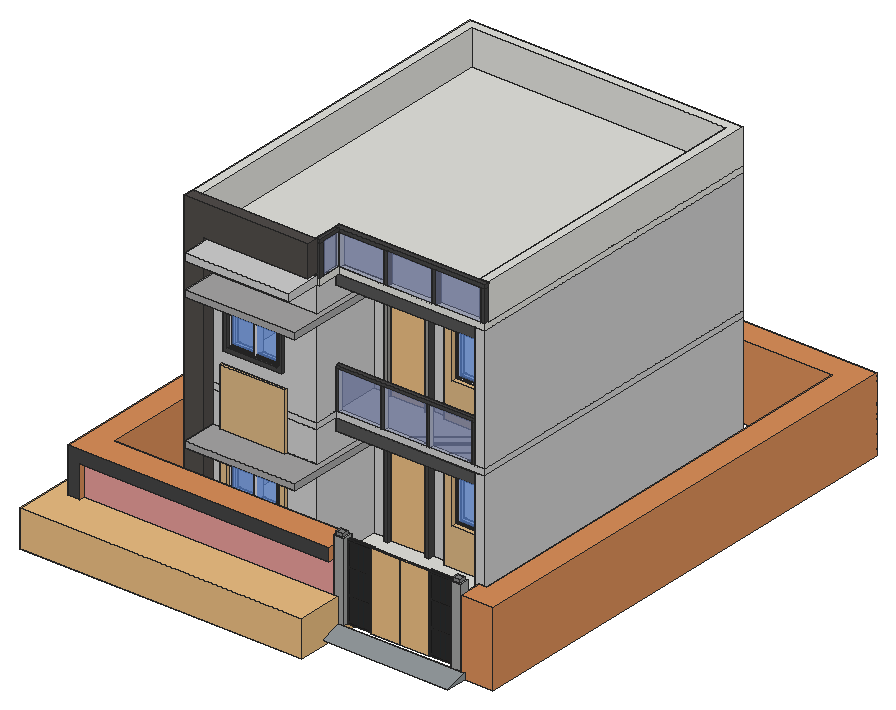
# SketchUp Ruby script. Lengths in inches.
U = 1.inch
M = Sketchup.active_model
def pt(a) = Geom::Point3d.new(a.map { |v| v * U })
def face(e, loops, mat)
  f = e.add_face(loops[0].map { |a| pt(a) })
  loops[1..].each { |l| e.add_face(l.map { |a| pt(a) }).erase! }
  f.material = f.back_material = mat if mat
  f
end
# faces: each face lists its corners as indices into pts; further lists are holes
def faces(e, pts, list, mat = nil) = list.each { |f| face(e, (f[0].is_a?(Array) ? f : [f]).map { |l| l.map { |i| pts[i] } }, mat) }
# xy, xz, yz: faces in a plane at the given z, y or x. An outline is a flat list of corners, or four numbers for a rectangle; further outlines are holes
def ring(l) = l.size == 4 ? [[l[0], l[1]], [l[2], l[1]], [l[2], l[3]], [l[0], l[3]]] : l.each_slice(2).to_a
def flat(e, list, mat, &to3) = list.each { |f| face(e, (f[0].is_a?(Array) ? f : [f]).map { |l| ring(l).map { |u, v| to3.(u, v) } }, mat) }
def xy(e, z, list, mat = nil) = flat(e, list, mat) { |x, y| [x, y, z] }
def xz(e, y, list, mat = nil) = flat(e, list, mat) { |x, z| [x, y, z] }
def yz(e, x, list, mat = nil) = flat(e, list, mat) { |y, z| [x, y, z] }
def lines(e, pts, list) = list.each { |a, b| e.add_line(pt(pts[a]), pt(pts[b])) }
# prism: a flat outline (further loops are holes) pulled along v
def prism(e, loops, v, mat = nil)
  f = face(e, loops, mat); d = Geom::Vector3d.new(v.map { |x| x * U })
  f.pushpull(f.normal.samedirection?(d) ? d.length : -d.length)
end
def box(e, o, s, mat = nil) = prism(e, [[o, [o[0] + s[0], o[1], o[2]], [o[0] + s[0], o[1] + s[1], o[2]], [o[0], o[1] + s[1], o[2]]]], [0, 0, s[2]], mat)
def at(x, y, z, deg = 0) = Geom::Transformation.translation(pt([x, y, z])) * Geom::Transformation.rotation(ORIGIN, Z_AXIS, deg.degrees)
def axes(o, x, y, z) = Geom::Transformation.new([*x, 0, *y, 0, *z, 0, *pt(o).to_a, 1])
def part(name) = M.definitions.add(name)
# library, detail: a bought-in or finely detailed component or shape, given as its bounding box
def library(name, o, s) = part(name).tap { |d| box(d.entities, o, s) }
def detail(e, o, s) = box(e.add_group.entities, o, s)
def put(e, d, t, mat = nil) = e.add_instance(d, t).tap { |i| i.material = mat if mat }
def group(e, t, mat = nil) = e.add_group.tap { |g| g.transformation = t; g.material = mat if mat }.entities
root = M.entities
M.materials.add("18776129-polished-granite-texture-in-whites-grays-and-blacks").color = [192, 192, 186]
M.materials.add("Lisanne_Eraser").color = [146, 152, 155]
M.materials.add("Stone_A_200cm").color = [133, 133, 133]
M.materials.add("Stone_A_200cmgach trang tri").color = [160, 161, 160]
M.materials.add("THEPDEN").color = [42, 49, 51]
M.materials.add("[Beadboard]").color = [218, 143, 90]
M.materials.add("[Brick Basket]").color = [230, 156, 152]
M.materials.add("[Carrera Marble]").color = [207, 207, 207]
M.materials.add("[Cladding Siding White]").color = [207, 207, 207]
M.materials.add("[Granite Dark Gray]").color = [69, 68, 68]
M.materials.add("[Granite Light Gray]").color = [149, 148, 144]
M.materials.add("[Metal Rusted]").color = [184, 117, 91]
M.materials.add("[Metal Silver]").color = [234, 233, 238]
M.materials.add("[Roofing Shingles GAF Estates]").color = [81, 77, 74]
M.materials.add("[Stone Vein Gray]").color = [166, 165, 165]
M.materials.add("[Suede Blue]").color = [50, 57, 70]
M.materials.add("[Suede Dark Gray]").color = [85, 85, 85]
M.materials.add("[Translucent Glass Blue]").color = [100, 149, 237]
M.materials["[Translucent Glass Blue]"].alpha = 0.5
M.materials.add("[Translucent Glass Sky Reflection]").color = [126, 138, 183]
M.materials["[Translucent Glass Sky Reflection]"].alpha = 0.52
M.materials.add("[Wallpaper Stripe]").color = [222, 185, 133]
M.materials.add("sat son den1").color = [33, 33, 33]
c1 = part("Component\#28")
box(c1.entities,[0,0,0],[7.875,7.875,3.9375],"Stone_A_200cm")
c2 = library("Group\#58",[-9.3,-11.72,-5.59],[177.13,38.12,35])
c3 = part("Vertical slat panel")
g1 = group(c3.entities,at(21.95,0,0))
box(g1,[0,0,0],[0.79,1.57,29.73],"THEPDEN")
g2 = group(c3.entities,at(5.49,0,0))
box(g2,[0,0,0],[0.79,1.57,29.73],"THEPDEN")
g3 = group(c3.entities,at(10.98,0,0))
box(g3,[0,0,0],[0.79,1.57,29.73],"THEPDEN")
g4 = group(c3.entities,at(7.84,0.79,0,-90))
box(g4,[0,0,0],[0.79,1.57,29.73],"THEPDEN")
g5 = group(c3.entities,at(13.33,0.79,0,-90))
box(g5,[0,0,0],[0.79,1.57,29.73],"THEPDEN")
g6 = group(c3.entities,at(2.35,0.79,0,-90))
box(g6,[0,0,0],[0.79,1.57,29.73],"THEPDEN")
g7 = group(c3.entities,at(18.8125,0.79,0,-90))
box(g7,[0,0,0],[0.79,1.57,29.73],"THEPDEN")
g8 = group(c3.entities,at(16.46,0,0))
box(g8,[0,0,0],[0.79,1.57,29.73],"THEPDEN")
g9 = group(c3.entities,at(24.3,0.79,0,-90))
box(g9,[0,0,0],[0.79,1.57,29.73],"THEPDEN")
c4 = part("Slatted gate leaf")
put(c4.entities,c3,axes([24.84,1.79,-51.33],[1.0302,0,0],[0,1,0],[0,0,0.84297]))
put(c4.entities,c3,axes([24.84,1.79,-104.14],[1.0302,0,0],[0,1,0],[0,0,0.82146]))
put(c4.entities,c3,axes([24.84,1.79,-78.28],[1.0302,0,0],[0,1,0],[0,0,0.8582]))
g10 = group(c4.entities,at(34.94,4.25,0))
xy(g10,-105.55,[[-10.84,-4.25,19.38,0]],"sat son den1")
xy(g10,-103.49,[[-8.39,-4.25,16.93,0]],"sat son den1")
xy(g10,-79.72,[[-9.2,-4.25,-8.39,0],[-8.39,-4.25,16.93,0],[16.93,-4.25,17.74,0]],"sat son den1")
xy(g10,-79.24,[[-10.37,-4.25,-9.2,0],[17.74,-4.25,18.92,0]],"sat son den1")
xy(g10,-78.77,[[-10.37,-4.25,-9.2,0],[17.74,-4.25,18.92,0]],"sat son den1")
xy(g10,-78.28,[[-9.2,-4.25,-8.39,0],[-8.39,-4.25,16.93,0],[16.93,-4.25,17.74,0]],"sat son den1")
xy(g10,-52.77,[[-9.2,-4.25,-8.39,0],[-8.39,-4.25,16.93,0],[16.93,-4.25,17.74,0]],"sat son den1")
xy(g10,-52.28,[[-10.37,-4.25,-9.2,0],[17.74,-4.25,18.92,0]],"sat son den1")
xy(g10,-51.82,[[-10.37,-4.25,-9.2,0],[17.74,-4.25,18.92,0]],"sat son den1")
xy(g10,-51.33,[[-9.2,-4.25,-8.39,0],[-8.39,-4.25,16.93,0],[16.93,-4.25,17.74,0]],"sat son den1")
xy(g10,-26.92,[[-8.39,-4.25,16.93,0]],"sat son den1")
xy(g10,-26.27,[[-10.37,-4.25,-8.39,0],[16.93,-4.25,17.74,0]],"sat son den1")
xy(g10,-25.33,[[17.74,-4.25,18.92,0]],"sat son den1")
xy(g10,-24.87,[[-10.84,-4.25,-10.37,0],[-10.37,-4.25,18.92,0],[18.92,-4.25,19.38,0]],"sat son den1")
xz(g10,-4.25,[[-10.84,-105.55,19.38,-105.55,19.38,-24.87,18.92,-24.87,18.92,-25.33,17.74,-25.33,17.74,-26.27,16.93,-26.27,16.93,-51.33,17.74,-51.33,17.74,-51.82,18.92,-51.82,18.92,-52.28,17.74,-52.28,17.74,-52.77,16.93,-52.77,16.93,-78.28,17.74,-78.28,17.74,-78.77,18.92,-78.77,18.92,-79.24,17.74,-79.24,17.74,-79.72,16.93,-79.72,16.93,-103.49,-8.39,-103.49,-8.39,-79.72,-9.2,-79.72,-9.2,-79.24,-10.37,-79.24,-10.37,-78.77,-9.2,-78.77,-9.2,-78.28,-8.39,-78.28,-8.39,-52.77,-9.2,-52.77,-9.2,-52.28,-10.37,-52.28,-10.37,-51.82,-9.2,-51.82,-9.2,-51.33,-8.39,-51.33,-8.39,-26.27,-10.37,-26.27,-10.37,-24.87,-10.84,-24.87],[-9.2,-79.72,17.74,-79.72,17.74,-79.24,18.92,-79.24,18.92,-78.77,17.74,-78.77,17.74,-78.28,-9.2,-78.28,-9.2,-78.77,-10.37,-78.77,-10.37,-79.24,-9.2,-79.24],[-9.2,-52.77,17.74,-52.77,17.74,-52.28,18.92,-52.28,18.92,-51.82,17.74,-51.82,17.74,-51.33,-9.2,-51.33,-9.2,-51.82,-10.37,-51.82,-10.37,-52.28,-9.2,-52.28],[-8.39,-26.92,16.93,-26.92,16.93,-26.27,17.74,-26.27,17.74,-25.33,18.92,-25.33,18.92,-24.87,-10.37,-24.87,-10.37,-26.27,-8.39,-26.27]],"sat son den1")
xz(g10,0,[[-10.84,-105.55,-10.84,-24.87,-10.37,-24.87,-10.37,-26.27,-8.39,-26.27,-8.39,-51.33,-9.2,-51.33,-9.2,-51.82,-10.37,-51.82,-10.37,-52.28,-9.2,-52.28,-9.2,-52.77,-8.39,-52.77,-8.39,-78.28,-9.2,-78.28,-9.2,-78.77,-10.37,-78.77,-10.37,-79.24,-9.2,-79.24,-9.2,-79.72,-8.39,-79.72,-8.39,-103.49,16.93,-103.49,16.93,-79.72,17.74,-79.72,17.74,-79.24,18.92,-79.24,18.92,-78.77,17.74,-78.77,17.74,-78.28,16.93,-78.28,16.93,-52.77,17.74,-52.77,17.74,-52.28,18.92,-52.28,18.92,-51.82,17.74,-51.82,17.74,-51.33,16.93,-51.33,16.93,-26.27,17.74,-26.27,17.74,-25.33,18.92,-25.33,18.92,-24.87,19.38,-24.87,19.38,-105.55],[-9.2,-79.72,-9.2,-79.24,-10.37,-79.24,-10.37,-78.77,-9.2,-78.77,-9.2,-78.28,17.74,-78.28,17.74,-78.77,18.92,-78.77,18.92,-79.24,17.74,-79.24,17.74,-79.72],[-9.2,-52.77,-9.2,-52.28,-10.37,-52.28,-10.37,-51.82,-9.2,-51.82,-9.2,-51.33,17.74,-51.33,17.74,-51.82,18.92,-51.82,18.92,-52.28,17.74,-52.28,17.74,-52.77],[-8.39,-26.92,-8.39,-26.27,-10.37,-26.27,-10.37,-24.87,18.92,-24.87,18.92,-25.33,17.74,-25.33,17.74,-26.27,16.93,-26.27,16.93,-26.92]],"sat son den1")
yz(g10,-10.84,[[-4.25,-105.55,0,-24.87]],"sat son den1")
yz(g10,-10.37,[[-4.25,-79.24,0,-78.77],[-4.25,-52.28,0,-51.82],[-4.25,-26.27,0,-24.87]],"sat son den1")
yz(g10,-9.2,[[-4.25,-79.72,0,-79.24],[-4.25,-78.77,0,-78.28],[-4.25,-52.77,0,-52.28],[-4.25,-51.82,0,-51.33]],"sat son den1")
yz(g10,-8.39,[[-4.25,-103.49,0,-79.72],[-4.25,-78.28,0,-52.77],[-4.25,-51.33,0,-26.92],[-4.25,-26.92,0,-26.27]],"sat son den1")
yz(g10,16.93,[[-4.25,-103.49,0,-79.72],[-4.25,-78.28,0,-52.77],[-4.25,-51.33,0,-26.92],[-4.25,-26.92,0,-26.27]],"sat son den1")
yz(g10,17.74,[[-4.25,-79.72,0,-79.24],[-4.25,-78.77,0,-78.28],[-4.25,-52.77,0,-52.28],[-4.25,-51.82,0,-51.33],[-4.25,-26.27,0,-25.33]],"sat son den1")
yz(g10,18.92,[[-4.25,-79.24,0,-78.77],[-4.25,-52.28,0,-51.82],[-4.25,-25.33,0,-24.87]],"sat son den1")
yz(g10,19.38,[[-4.25,-105.55,0,-24.87]],"sat son den1")
c5 = library("Group\#45",[0,-0.15,0],[31.47,2.91,94.32])
c6 = library("Group\#35",[0,-0.15,0],[31.47,2.91,94.32])
c7 = part("cong+trinh+1")
put(c7.entities,c1,axes([-761.28,-1219.33,75.2],[0.82267,0,0],[0,0.76,0],[0,0,0.75]))
put(c7.entities,c1,axes([-647.9,-1219.33,75.2],[0.82267,0,0],[0,0.76,0],[0,0,0.75]))
g11 = group(c7.entities,at(614.78,209.1,-17.8125))
g12 = group(g11,at(-1250.68,-1449.6,11.8125),"18776129-polished-granite-texture-in-whites-grays-and-blacks")
prism(g12,[[[-132.06,19.69,5.91],[-132.06,19.69,0],[-132.06,0,0]]],[132.06,0,0],"Lisanne_Eraser")
put(c7.entities,c2,axes([-1016.9,-1244.91,-6],[1.5402,0,0],[0,1.68,0],[0,0,1]))
g13 = group(c7.entities,at(-649.52,-1220.82,-0.09))
box(g13,[0,0,0],[9.72,8.98,75.3],"Stone_A_200cmgach trang tri")
g14 = group(c7.entities,at(-762.9,-1220.82,-0.09))
box(g14,[0,0,0],[9.72,8.98,75.3],"Stone_A_200cmgach trang tri")
g15 = group(c7.entities,at(-753.18,-1217.23,-0.09))
put(g15,c4,axes([60.26,3.95,-22.7],[0.79856,0,0],[0,-0.76,0],[0,0,-0.913]))
put(g15,c4,axes([-19.25,3.95,-22.7],[0.79856,0,0],[0,-0.76,0],[0,0,-0.913]))
put(g15,c5,axes([24.03,0.12,0],[0.88335,0,0],[0,0.76,0],[0,0,0.78261]),"THEPDEN")
put(g15,c6,axes([79.62,0.12,0],[-0.88335,0,0],[0,0.76,0],[0,0,0.78261]))
c8 = part("Group4\#2")
box(c8.entities,[1.02,-2.16,1.02],[46.66,0.63,45.96])
c9 = part("Group\#3")
g16 = group(c9.entities,at(48.7,0,0,180),"[Metal Silver]")
xy(g16,0,[[0,-9,23.52,0],[23.52,-9,25.18,0],[25.18,-9,48.7,0]])
xy(g16,0.83,[[0.83,-8.93,23.52,-4.61],[25.18,-8.93,47.875,-4.61]])
xy(g16,1.02,[[1.02,-3.3125,23.52,-2.16],[23.52,-3.3125,25.18,-2.16],[25.18,-3.3125,47.68,-2.16]])
xy(g16,1.61,[[1.61,-2.16,23.52,-1.8],[25.18,-2.16,47.09,-1.8]])
xy(g16,1.65,[[1.65,-3.46,23.52,-3.3125],[25.18,-3.46,47.05,-3.3125]])
xy(g16,46.35,[[1.65,-3.46,23.52,-3.3125],[25.18,-3.46,47.05,-3.3125]])
xy(g16,46.39,[[1.61,-2.16,23.52,-1.8],[25.18,-2.16,47.09,-1.8]])
xy(g16,46.98,[[1.02,-3.3125,23.52,-2.16],[23.52,-3.3125,25.18,-2.16],[25.18,-3.3125,47.68,-2.16]])
xy(g16,47.17,[[0.83,-8.93,23.52,-4.61],[25.18,-8.93,47.875,-4.61]])
xy(g16,48,[[0,-9,23.52,0],[23.52,-9,25.18,0],[25.18,-9,48.7,0]])
xz(g16,-9.07,[[0.04,0.04,23.52,0.04,23.52,0.75,0.75,0.75,0.75,47.25,23.52,47.25,23.52,47.96,0.04,47.96],[23.52,0.04,25.18,47.96],[25.18,0.04,48.66,0.04,48.66,47.96,25.18,47.96,25.18,47.25,47.95,47.25,47.95,0.75,25.18,0.75]])
xz(g16,-4.61,[[0.83,0.83,23.52,0.83,23.52,1.5,1.5,1.5,1.5,46.5,23.52,46.5,23.52,47.17,0.83,47.17],[25.18,0.83,47.875,0.83,47.875,47.17,25.18,47.17,25.18,46.5,47.21,46.5,47.21,1.5,25.18,1.5]])
xz(g16,-3.3125,[[1.02,1.02,1.02,46.98,23.52,46.98,23.52,46.35,1.65,46.35,1.65,1.65,23.52,1.65,23.52,1.02],[23.52,1.02,25.18,46.98],[25.18,1.02,25.18,1.65,47.05,1.65,47.05,46.35,25.18,46.35,25.18,46.98,47.68,46.98,47.68,1.02]])
xz(g16,-2.16,[[1.02,1.02,23.52,1.02,23.52,1.61,1.61,1.61,1.61,46.39,23.52,46.39,23.52,46.98,1.02,46.98],[23.52,1.02,25.18,46.98],[25.18,1.02,47.68,1.02,47.68,46.98,25.18,46.98,25.18,46.39,47.09,46.39,47.09,1.61,25.18,1.61]])
xz(g16,-1.8,[[0.83,0.83,0.83,47.17,23.52,47.17,23.52,46.39,1.61,46.39,1.61,1.61,23.52,1.61,23.52,0.83],[25.18,0.83,25.18,1.61,47.09,1.61,47.09,46.39,25.18,46.39,25.18,47.17,47.875,47.17,47.875,0.83]])
xz(g16,-0.36,[[0.59,0.59,0.59,47.41,23.52,47.41,23.52,47.21,0.79,47.21,0.79,0.79,23.52,0.79,23.52,0.59],[25.18,0.59,25.18,0.79,47.91,0.79,47.91,47.21,25.18,47.21,25.18,47.41,48.11,47.41,48.11,0.59]])
xz(g16,0,[[0,0,0,48,23.52,48,23.52,47.61,0.39,47.61,0.39,0.39,23.52,0.39,23.52,0],[23.52,0,25.18,48],[25.18,0,25.18,0.39,48.31,0.39,48.31,47.61,25.18,47.61,25.18,48,48.7,48,48.7,0]])
yz(g16,0,[[-9,0,0,48]])
yz(g16,0.83,[[-8.93,0.83,-4.61,47.17]])
yz(g16,1.02,[[-3.3125,1.02,-2.16,46.98]])
yz(g16,1.61,[[-2.16,1.61,-1.8,46.39]])
yz(g16,1.65,[[-3.46,1.65,-3.3125,46.35]])
yz(g16,23.52,[[-9,0,0,0,0,0.39,-0.36,0.59,-0.36,0.79,-1.8,0.83,-1.8,1.61,-2.16,1.61,-2.16,1.02,-3.3125,1.02,-3.3125,1.65,-3.46,1.65,-4.61,1.5,-4.61,0.83,-8.93,0.83,-9.07,0.75,-9.07,0.04],[[-9,0,-9.07,0.04,-9.07,47.96,-9,48,0,48,0,0],[-3.3125,1.02,-2.16,46.98]],[-3.46,46.35,-3.3125,46.35,-3.3125,46.98,-2.16,46.98,-2.16,46.39,-1.8,46.39,-1.8,47.17,-0.36,47.21,-0.36,47.41,0,47.61,0,48,-9,48,-9.07,47.96,-9.07,47.25,-8.93,47.17,-4.61,47.17,-4.61,46.5]])
yz(g16,25.18,[[-9,0,-9.07,0.04,-9.07,0.75,-8.93,0.83,-4.61,0.83,-4.61,1.5,-3.46,1.65,-3.3125,1.65,-3.3125,1.02,-2.16,1.02,-2.16,1.61,-1.8,1.61,-1.8,0.83,-0.36,0.79,-0.36,0.59,0,0.39,0,0],[[-9,0,0,0,0,48,-9,48,-9.07,47.96,-9.07,0.04],[-3.3125,1.02,-2.16,46.98]],[-3.46,46.35,-4.61,46.5,-4.61,47.17,-8.93,47.17,-9.07,47.25,-9.07,47.96,-9,48,0,48,0,47.61,-0.36,47.41,-0.36,47.21,-1.8,47.17,-1.8,46.39,-2.16,46.39,-2.16,46.98,-3.3125,46.98,-3.3125,46.35]])
yz(g16,47.05,[[-3.46,1.65,-3.3125,46.35]])
yz(g16,47.09,[[-2.16,1.61,-1.8,46.39]])
yz(g16,47.68,[[-3.3125,1.02,-2.16,46.98]])
yz(g16,47.875,[[-8.93,0.83,-4.61,47.17]])
yz(g16,48.7,[[-9,0,0,48]])
p = [[23.52,-9,0],[23.52,-9.07,0.04],[0.04,-9.07,0.04],[0,-9,0],[0.04,-9.07,47.96],[0,-9,48],
  [25.18,-9,0],[25.18,-9.07,0.04],[48.7,-9,0],[48.66,-9.07,0.04],[48.7,-9,48],[48.66,-9.07,47.96],
  [23.52,-0.36,0.59],[23.52,0,0.39],[0.39,0,0.39],[0.59,-0.36,0.59],[0.39,0,47.61],[0.59,-0.36,47.41],
  [25.18,0,0.39],[25.18,-0.36,0.59],[48.11,-0.36,0.59],[48.31,0,0.39],[48.11,-0.36,47.41],[48.31,0,47.61],
  [23.52,-9.07,0.75],[23.52,-8.93,0.83],[0.83,-8.93,0.83],[0.75,-9.07,0.75],[0.83,-8.93,47.17],[0.75,-9.07,47.25],
  [25.18,-8.93,0.83],[25.18,-9.07,0.75],[47.95,-9.07,0.75],[47.875,-8.93,0.83],[47.95,-9.07,47.25],[47.875,-8.93,47.17],
  [23.52,-1.8,0.83],[23.52,-0.36,0.79],[0.79,-0.36,0.79],[0.83,-1.8,0.83],[0.79,-0.36,47.21],[0.83,-1.8,47.17],
  [25.18,-0.36,0.79],[25.18,-1.8,0.83],[47.875,-1.8,0.83],[47.91,-0.36,0.79],[47.875,-1.8,47.17],[47.91,-0.36,47.21],
  [23.52,-4.61,1.5],[23.52,-3.46,1.65],[1.65,-3.46,1.65],[1.5,-4.61,1.5],[1.65,-3.46,46.35],[1.5,-4.61,46.5],
  [25.18,-3.46,1.65],[25.18,-4.61,1.5],[47.21,-4.61,1.5],[47.05,-3.46,1.65],[47.21,-4.61,46.5],[47.05,-3.46,46.35],
  [23.52,-3.46,46.35],[23.52,-4.61,46.5],[25.18,-4.61,46.5],[25.18,-3.46,46.35],[23.52,-8.93,47.17],[23.52,-9.07,47.25],
  [25.18,-9.07,47.25],[25.18,-8.93,47.17],[23.52,-0.36,47.21],[23.52,-1.8,47.17],[25.18,-1.8,47.17],[25.18,-0.36,47.21],
  [23.52,0,47.61],[23.52,-0.36,47.41],[25.18,-0.36,47.41],[25.18,0,47.61],[23.52,-9.07,47.96],[23.52,-9,48],
  [25.18,-9.07,47.96],[25.18,-9,48]]
faces(g16,p,[[0,1,2,3],[3,2,4,5],[6,7,1,0],[7,6,8,9],[9,8,10,11],[12,13,14,15],[15,14,16,17],[18,19,20,21],
  [21,20,22,23],[24,25,26,27],[27,26,28,29],[30,31,32,33],[33,32,34,35],[36,37,38,39],[39,38,40,41],[42,43,44,45],
  [45,44,46,47],[48,49,50,51],[51,50,52,53],[54,55,56,57],[57,56,58,59],[53,52,60,61],[59,58,62,63],[29,28,64,65],
  [35,34,66,67],[41,40,68,69],[47,46,70,71],[17,16,72,73],[23,22,74,75],[5,4,76,77],[78,79,77,76],[11,10,79,78]])
put(c9.entities,c8,at(48.7,0,0,180),"[Translucent Glass Blue]")
c10 = part("Group7\#2")
box(c10.entities,[1.02,-2.16,1.02],[45.96,0.63,45.96])
c11 = part("Group\#5")
put(c11.entities,c10,at(48,0,0,180),"[Translucent Glass Blue]")
g17 = group(c11.entities,at(48,0,0,180),"[Metal Silver]")
xy(g17,0,[[0,-9,23.17,0],[23.17,-9,24.83,0],[24.83,-9,48,0]])
xy(g17,0.83,[[0.83,-8.93,23.17,-4.61],[24.83,-8.93,47.17,-4.61]])
xy(g17,1.02,[[1.02,-3.3125,23.17,-2.16],[23.17,-3.3125,24.83,-2.16],[24.83,-3.3125,46.98,-2.16]])
xy(g17,1.61,[[1.61,-2.16,23.17,-1.8],[24.83,-2.16,46.39,-1.8]])
xy(g17,1.65,[[1.65,-3.46,23.17,-3.3125],[24.83,-3.46,46.35,-3.3125]])
xy(g17,46.35,[[1.65,-3.46,23.17,-3.3125],[24.83,-3.46,46.35,-3.3125]])
xy(g17,46.39,[[1.61,-2.16,23.17,-1.8],[24.83,-2.16,46.39,-1.8]])
xy(g17,46.98,[[1.02,-3.3125,23.17,-2.16],[23.17,-3.3125,24.83,-2.16],[24.83,-3.3125,46.98,-2.16]])
xy(g17,47.17,[[0.83,-8.93,23.17,-4.61],[24.83,-8.93,47.17,-4.61]])
xy(g17,48,[[0,-9,23.17,0],[23.17,-9,24.83,0],[24.83,-9,48,0]])
xz(g17,-9.07,[[0.04,0.04,23.17,0.04,23.17,0.75,0.75,0.75,0.75,47.25,23.17,47.25,23.17,47.96,0.04,47.96],[23.17,0.04,24.83,47.96],[24.83,0.04,47.96,0.04,47.96,47.96,24.83,47.96,24.83,47.25,47.25,47.25,47.25,0.75,24.83,0.75]])
xz(g17,-4.61,[[0.83,0.83,23.17,0.83,23.17,1.5,1.5,1.5,1.5,46.5,23.17,46.5,23.17,47.17,0.83,47.17],[24.83,0.83,47.17,0.83,47.17,47.17,24.83,47.17,24.83,46.5,46.5,46.5,46.5,1.5,24.83,1.5]])
xz(g17,-3.3125,[[1.02,1.02,1.02,46.98,23.17,46.98,23.17,46.35,1.65,46.35,1.65,1.65,23.17,1.65,23.17,1.02],[23.17,1.02,24.83,46.98],[24.83,1.02,24.83,1.65,46.35,1.65,46.35,46.35,24.83,46.35,24.83,46.98,46.98,46.98,46.98,1.02]])
xz(g17,-2.16,[[1.02,1.02,23.17,1.02,23.17,1.61,1.61,1.61,1.61,46.39,23.17,46.39,23.17,46.98,1.02,46.98],[23.17,1.02,24.83,46.98],[24.83,1.02,46.98,1.02,46.98,46.98,24.83,46.98,24.83,46.39,46.39,46.39,46.39,1.61,24.83,1.61]])
xz(g17,-1.8,[[0.83,0.83,0.83,47.17,23.17,47.17,23.17,46.39,1.61,46.39,1.61,1.61,23.17,1.61,23.17,0.83],[24.83,0.83,24.83,1.61,46.39,1.61,46.39,46.39,24.83,46.39,24.83,47.17,47.17,47.17,47.17,0.83]])
xz(g17,-0.36,[[0.59,0.59,0.59,47.41,23.17,47.41,23.17,47.21,0.79,47.21,0.79,0.79,23.17,0.79,23.17,0.59],[24.83,0.59,24.83,0.79,47.21,0.79,47.21,47.21,24.83,47.21,24.83,47.41,47.41,47.41,47.41,0.59]])
xz(g17,0,[[0,0,0,48,23.17,48,23.17,47.61,0.39,47.61,0.39,0.39,23.17,0.39,23.17,0],[23.17,0,24.83,48],[24.83,0,24.83,0.39,47.61,0.39,47.61,47.61,24.83,47.61,24.83,48,48,48,48,0]])
yz(g17,0,[[-9,0,0,48]])
yz(g17,0.83,[[-8.93,0.83,-4.61,47.17]])
yz(g17,1.02,[[-3.3125,1.02,-2.16,46.98]])
yz(g17,1.61,[[-2.16,1.61,-1.8,46.39]])
yz(g17,1.65,[[-3.46,1.65,-3.3125,46.35]])
yz(g17,23.17,[[-9,0,0,0,0,0.39,-0.36,0.59,-0.36,0.79,-1.8,0.83,-1.8,1.61,-2.16,1.61,-2.16,1.02,-3.3125,1.02,-3.3125,1.65,-3.46,1.65,-4.61,1.5,-4.61,0.83,-8.93,0.83,-9.07,0.75,-9.07,0.04],[[-9,0,-9.07,0.04,-9.07,47.96,-9,48,0,48,0,0],[-3.3125,1.02,-2.16,46.98]],[-3.46,46.35,-3.3125,46.35,-3.3125,46.98,-2.16,46.98,-2.16,46.39,-1.8,46.39,-1.8,47.17,-0.36,47.21,-0.36,47.41,0,47.61,0,48,-9,48,-9.07,47.96,-9.07,47.25,-8.93,47.17,-4.61,47.17,-4.61,46.5]])
yz(g17,24.83,[[-9,0,-9.07,0.04,-9.07,0.75,-8.93,0.83,-4.61,0.83,-4.61,1.5,-3.46,1.65,-3.3125,1.65,-3.3125,1.02,-2.16,1.02,-2.16,1.61,-1.8,1.61,-1.8,0.83,-0.36,0.79,-0.36,0.59,0,0.39,0,0],[[-9,0,0,0,0,48,-9,48,-9.07,47.96,-9.07,0.04],[-3.3125,1.02,-2.16,46.98]],[-3.46,46.35,-4.61,46.5,-4.61,47.17,-8.93,47.17,-9.07,47.25,-9.07,47.96,-9,48,0,48,0,47.61,-0.36,47.41,-0.36,47.21,-1.8,47.17,-1.8,46.39,-2.16,46.39,-2.16,46.98,-3.3125,46.98,-3.3125,46.35]])
yz(g17,46.35,[[-3.46,1.65,-3.3125,46.35]])
yz(g17,46.39,[[-2.16,1.61,-1.8,46.39]])
yz(g17,46.98,[[-3.3125,1.02,-2.16,46.98]])
yz(g17,47.17,[[-8.93,0.83,-4.61,47.17]])
yz(g17,48,[[-9,0,0,48]])
p = [[23.17,-9,0],[23.17,-9.07,0.04],[0.04,-9.07,0.04],[0,-9,0],[0.04,-9.07,47.96],[0,-9,48],
  [24.83,-9,0],[24.83,-9.07,0.04],[48,-9,0],[47.96,-9.07,0.04],[48,-9,48],[47.96,-9.07,47.96],
  [23.17,-0.36,0.59],[23.17,0,0.39],[0.39,0,0.39],[0.59,-0.36,0.59],[0.39,0,47.61],[0.59,-0.36,47.41],
  [24.83,0,0.39],[24.83,-0.36,0.59],[47.41,-0.36,0.59],[47.61,0,0.39],[47.41,-0.36,47.41],[47.61,0,47.61],
  [23.17,-9.07,0.75],[23.17,-8.93,0.83],[0.83,-8.93,0.83],[0.75,-9.07,0.75],[0.83,-8.93,47.17],[0.75,-9.07,47.25],
  [24.83,-8.93,0.83],[24.83,-9.07,0.75],[47.25,-9.07,0.75],[47.17,-8.93,0.83],[47.25,-9.07,47.25],[47.17,-8.93,47.17],
  [23.17,-1.8,0.83],[23.17,-0.36,0.79],[0.79,-0.36,0.79],[0.83,-1.8,0.83],[0.79,-0.36,47.21],[0.83,-1.8,47.17],
  [24.83,-0.36,0.79],[24.83,-1.8,0.83],[47.17,-1.8,0.83],[47.21,-0.36,0.79],[47.17,-1.8,47.17],[47.21,-0.36,47.21],
  [23.17,-4.61,1.5],[23.17,-3.46,1.65],[1.65,-3.46,1.65],[1.5,-4.61,1.5],[1.65,-3.46,46.35],[1.5,-4.61,46.5],
  [24.83,-3.46,1.65],[24.83,-4.61,1.5],[46.5,-4.61,1.5],[46.35,-3.46,1.65],[46.5,-4.61,46.5],[46.35,-3.46,46.35],
  [23.17,-3.46,46.35],[23.17,-4.61,46.5],[24.83,-4.61,46.5],[24.83,-3.46,46.35],[23.17,-8.93,47.17],[23.17,-9.07,47.25],
  [24.83,-9.07,47.25],[24.83,-8.93,47.17],[23.17,-0.36,47.21],[23.17,-1.8,47.17],[24.83,-1.8,47.17],[24.83,-0.36,47.21],
  [23.17,0,47.61],[23.17,-0.36,47.41],[24.83,-0.36,47.41],[24.83,0,47.61],[23.17,-9.07,47.96],[23.17,-9,48],
  [24.83,-9.07,47.96],[24.83,-9,48]]
faces(g17,p,[[0,1,2,3],[3,2,4,5],[6,7,1,0],[7,6,8,9],[9,8,10,11],[12,13,14,15],[15,14,16,17],[18,19,20,21],
  [21,20,22,23],[24,25,26,27],[27,26,28,29],[30,31,32,33],[33,32,34,35],[36,37,38,39],[39,38,40,41],[42,43,44,45],
  [45,44,46,47],[48,49,50,51],[51,50,52,53],[54,55,56,57],[57,56,58,59],[53,52,60,61],[59,58,62,63],[29,28,64,65],
  [35,34,66,67],[41,40,68,69],[47,46,70,71],[17,16,72,73],[23,22,74,75],[5,4,76,77],[78,79,77,76],[11,10,79,78]])
c12 = library("Group\#6",[0,0,0],[36,10.47,82])
xy(root,252,[[193.125,81.54,195.0625,99.79],[195.875,99.79,238.71,104.85],[242.58,99.79,285.42,104.85],[289.29,99.79,332.125,104.85]])
xy(root,282.25,[[193.125,81.54,195.0625,99.79],[195.875,99.79,238.71,104.85],[242.58,99.79,285.42,104.85],[289.29,99.79,332.125,104.85]])
xz(root,81.54,[[193.125,252,195.0625,282.25]])
xz(root,99.79,[[193.125,252,195.0625,282.25]])
xz(root,99.79,[[195.875,252,238.71,282.25],[242.58,252,285.42,282.25],[289.29,252,332.125,282.25]],"[Translucent Glass Sky Reflection]")
xz(root,104.85,[[195.875,252,238.71,282.25],[242.58,252,285.42,282.25],[289.29,252,332.125,282.25]],"[Translucent Glass Sky Reflection]")
yz(root,193.125,[[81.54,252,99.79,282.25]],"[Translucent Glass Sky Reflection]")
yz(root,195.0625,[[81.54,252,99.79,282.25]],"[Translucent Glass Sky Reflection]")
yz(root,195.875,[[99.79,252,104.85,282.25]])
yz(root,238.71,[[99.79,252,104.85,282.25]])
yz(root,242.58,[[99.79,252,104.85,282.25]])
yz(root,285.42,[[99.79,252,104.85,282.25]])
yz(root,289.29,[[99.79,252,104.85,282.25]])
yz(root,332.125,[[99.79,252,104.85,282.25]])
put(root,c7,at(1016.57,1240.51,0))
g18 = group(root,at(72,42.73,-6))
xy(g18,6,[[0,23.125,19.3125,33.75]],"[Metal Rusted]")
xy(g18,115,[[120,57.0625,255,103.1875]],"[Suede Dark Gray]")
xy(g18,126,[[120,57.0625,255,103.1875]],"[Suede Blue]")
xy(g18,132,[[120,57.0625,123,57.0625,123,60.75,164,60.75,164,57.0625,167,57.0625,167,60.75,208,60.75,208,57.0625,211,57.0625,211,60.75,252,60.75,252,57.0625,255,57.0625,255,103.1875,120,103.1875]])
xy(g18,169.3125,[[123,57.0625,164,60.75],[167,57.0625,208,60.75],[211,57.0625,252,60.75]])
xy(g18,252,[[19.3125,0,120,33.75]],"[Carrera Marble]")
xy(g18,258,[[0,33.75,0,369.75,264,369.75,264,62.125,255,62.125,255,360.75,9,360.75,9,33.75]])
xy(g18,259,[[19.3125,0,120,33.75]],"[Carrera Marble]")
xy(g18,261.72,[[19.3125,23.125,120,33.75]],"[Metal Rusted]")
xy(g18,291.9375,[[0,33.75,9,33.75,9,360.75,255,360.75,255,62.125,264,62.125,264,369.75,0,369.75]])
xy(g18,291.9375,[[0,23.125,120,33.75]],"[Roofing Shingles GAF Estates]")
xz(g18,0,[[19.3125,252,120,259]],"[Carrera Marble]")
xz(g18,23.125,[[0,6,19.3125,6,19.3125,261.72,120,261.72,120,291.9375,0,291.9375]],"[Roofing Shingles GAF Estates]")
xz(g18,33.75,[[0,6,0,258,120,258,120,252,19.3125,252,19.3125,6],[0,258,9,291.9375],[19.3125,259,120,261.72]],"[Metal Rusted]")
xz(g18,33.75,[[9,258,9,291.9375,120,291.9375,120,261.72,19.3125,261.72,19.3125,259,120,259,120,258]],"[Roofing Shingles GAF Estates]")
xz(g18,57.0625,[[120,115,255,126]],"[Suede Dark Gray]")
xz(g18,57.0625,[[123,132,164,169.3125],[167,132,208,169.3125],[211,132,252,169.3125]],"[Translucent Glass Sky Reflection]")
xz(g18,60.75,[[123,132,164,169.3125],[167,132,208,169.3125],[211,132,252,169.3125]],"[Translucent Glass Sky Reflection]")
xz(g18,62.125,[[255,258,264,291.9375]])
xz(g18,103.1875,[[120,115,255,126]],"[Suede Blue]")
xz(g18,360.75,[[9,258,255,291.9375]])
xz(g18,369.75,[[0,258,264,291.9375]])
yz(g18,0,[[33.75,258,369.75,291.9375]])
yz(g18,0,[[23.125,6,33.75,291.9375]],"[Roofing Shingles GAF Estates]")
yz(g18,9,[[33.75,258,360.75,291.9375]])
yz(g18,19.3125,[[0,252,23.125,259]],"[Carrera Marble]")
yz(g18,19.3125,[[23.125,6,33.75,252],[23.125,259,33.75,261.72]],"[Roofing Shingles GAF Estates]")
yz(g18,120,[[0,252,33.75,259]],"[Carrera Marble]")
yz(g18,120,[[23.125,261.72,33.75,291.9375]],"[Roofing Shingles GAF Estates]")
yz(g18,120,[[57.0625,115,103.1875,126]],"[Suede Blue]")
yz(g18,123,[[57.0625,132,60.75,169.3125]])
yz(g18,164,[[57.0625,132,60.75,169.3125]])
yz(g18,167,[[57.0625,132,60.75,169.3125]])
yz(g18,208,[[57.0625,132,60.75,169.3125]])
yz(g18,211,[[57.0625,132,60.75,169.3125]])
yz(g18,252,[[57.0625,132,60.75,169.3125]])
yz(g18,255,[[62.125,258,360.75,291.9375]])
yz(g18,255,[[57.0625,115,103.1875,126]],"[Suede Blue]")
yz(g18,264,[[62.125,258,369.75,291.9375]])
g19 = group(g18,at(120,57.0625,169.3125),"[Granite Dark Gray]")
box(g19,[0,0,0],[135,3.6875,3])
g20 = group(g18,at(0,33.75,252))
xy(g20,6,[[0,0,123.0625,0,123.0625,23.3125,264,23.3125,264,336,0,336]])
xz(g20,0,[[0,0,123.0625,6]])
xz(g20,23.3125,[[123.0625,0,264,6]])
xz(g20,336,[[0,0,264,6]])
yz(g20,0,[[0,0,336,6]])
yz(g20,123.0625,[[0,0,23.3125,6]])
yz(g20,264,[[23.3125,0,336,6]])
g21 = group(g20,at(120,23.3125,0),"[Suede Dark Gray]")
box(g21,[0,0,-10.3125],[135,46.125,10.3125])
g22 = group(g18,at(0,33.75,6))
xy(g22,0,[[28.3,-2.625,28.3,0,0,0,0,336,264,336,264,23.3125,255,23.3125,255,64,191.875,64,191.875,69.4375,178,69.4375,178,64,174,64,174,78.4375,255,78.4375,255,327,9,327,9,9,111,9,111,78.4375,138,78.4375,138,64,134,64,134,69.4375,120,69.4375,120,0,91,0,91,-2.625]])
xy(g22,36,[[35.3,-2.625,84,9],[199.4375,64,247.4375,78.4375]],"[Wallpaper Stripe]")
xy(g22,82,[[138,64,174,78.4375]])
xy(g22,84,[[35.3,-2.625,84,9],[199.4375,64,247.4375,78.4375]],"[Wallpaper Stripe]")
xy(g22,86,[[134,64,178,69.4375]],"[Granite Dark Gray]")
xy(g22,109,[[191.875,64,255,69.4375]],"[Wallpaper Stripe]")
xy(g22,120,[[[0,0,120,0,120,69.4375,255,69.4375,255,23.3125,264,23.3125,264,336,0,336],[9,9,9,327,255,327,255,78.4375,111,78.4375,111,9]],[9,9,111,9,111,78.4375,255,78.4375,255,327,9,327]])
xy(g22,145.375,[[28.3,-2.625,91,0]],"[Wallpaper Stripe]")
xz(g22,-2.625,[[[28.3,0,91,145.375],[35.3,36,84,84]]],"[Wallpaper Stripe]")
xz(g22,0,[[28.3,120,91,145.375]])
xz(g22,0,[[0,0,28.3,120],[91,0,120,120]],"[Cladding Siding White]")
xz(g22,9,[[[9,0,111,120],[35.3,36,84,84]]])
xz(g22,23.3125,[[255,0,264,120]],"[Cladding Siding White]")
xz(g22,64,[[[191.875,0,255,109],[199.4375,36,247.4375,84]]],"[Wallpaper Stripe]")
xz(g22,69.4375,[[120,0,134,0,134,86,178,86,178,0,191.875,0,191.875,109,255,109,255,120,120,120]],"[Cladding Siding White]")
xz(g22,78.4375,[[[111,0,111,120,255,120,255,0,174,0,174,82,138,82,138,0],[199.4375,36,247.4375,84]]])
xz(g22,327,[[9,0,255,120]])
xz(g22,336,[[0,0,264,120]],"[Cladding Siding White]")
yz(g22,0,[[0,0,336,120]],"[Cladding Siding White]")
yz(g22,9,[[9,0,327,120]])
yz(g22,28.3,[[-2.625,0,0,145.375]],"[Wallpaper Stripe]")
yz(g22,35.3,[[-2.625,36,9,84]],"[Wallpaper Stripe]")
yz(g22,84,[[-2.625,36,9,84]],"[Wallpaper Stripe]")
yz(g22,91,[[-2.625,0,0,145.375]],"[Wallpaper Stripe]")
yz(g22,111,[[9,0,78.4375,120]])
yz(g22,120,[[0,0,69.4375,120]],"[Cladding Siding White]")
yz(g22,134,[[64,0,69.4375,86]],"[Granite Dark Gray]")
yz(g22,138,[[64,0,78.4375,82]],"[Granite Dark Gray]")
yz(g22,174,[[64,0,78.4375,82]],"[Granite Dark Gray]")
yz(g22,178,[[64,0,69.4375,86]],"[Granite Dark Gray]")
yz(g22,191.875,[[64,0,69.4375,109]],"[Wallpaper Stripe]")
yz(g22,199.4375,[[64,36,78.4375,84]],"[Wallpaper Stripe]")
yz(g22,247.4375,[[64,36,78.4375,84]],"[Wallpaper Stripe]")
yz(g22,255,[[78.4375,0,327,120]])
yz(g22,255,[[23.3125,0,23.3125,120,69.4375,120,69.4375,109,64,109,64,0]],"[Cladding Siding White]")
yz(g22,264,[[23.3125,0,336,120]],"[Cladding Siding White]")
put(g22,c9,at(35.3,0,36))
put(g22,c11,at(199.4375,69.4375,36))
put(g22,c12,at(138,67.97,0),"[Granite Dark Gray]")
g23 = group(g22,at(134,64,0),"[Granite Dark Gray]")
xz(g23,0,[[0,0,4,0,4,82,40,82,40,0,44,0,44,86,0,86]])
g24 = group(g18,at(0,33.75,0))
prism(g24,[[[264,336,0],[264,0,0],[120,0,0],[0,0,0],[0,336,0]]],[0,0,6])
g25 = group(g18,at(0,33.75,132))
xy(g25,0,[[0,0,0,336,264,336,264,23.3125,255,23.3125,255,64,191.875,64,191.875,69.4375,178,69.4375,178,64,174,64,174,78.4375,255,78.4375,255,327,9,327,9,9,111,9,111,78.4375,138,78.4375,138,64,134,64,134,69.4375,120,69.4375,120,0]])
xy(g25,32,[[31.3,-2.6875,88,0]],"[Granite Dark Gray]")
xy(g25,36,[[35.3,-2.6875,84,9]],"[Granite Dark Gray]")
xy(g25,36,[[199.4375,64,247.4375,78.4375]],"[Wallpaper Stripe]")
xy(g25,82,[[138,64,174,78.4375]])
xy(g25,84,[[35.3,-2.6875,84,9]])
xy(g25,84,[[199.4375,64,247.4375,78.4375]],"[Wallpaper Stripe]")
xy(g25,86,[[134,64,178,69.4375]],"[Granite Light Gray]")
xy(g25,88,[[31.3,-2.6875,88,0]],"[Granite Dark Gray]")
xy(g25,109,[[191.875,64,255,69.4375]],"[Wallpaper Stripe]")
xy(g25,120,[[[0,0,120,0,120,69.4375,264,69.4375,264,336,0,336],[9,9,9,327,255,327,255,78.4375,111,78.4375,111,9]],[9,9,111,9,111,78.4375,255,78.4375,255,327,9,327],[255,23.3125,264,69.4375]])
xz(g25,-2.6875,[[[31.3,32,88,88],[35.3,36,84,84]]],"[Granite Dark Gray]")
xz(g25,0,[[[0,0,120,120],[31.3,32,88,88]]],"[Cladding Siding White]")
xz(g25,9,[[[9,0,111,120],[35.3,36,84,84]]])
xz(g25,23.3125,[[255,0,264,120]],"[Cladding Siding White]")
xz(g25,64,[[[191.875,0,255,109],[199.4375,36,247.4375,84]]],"[Wallpaper Stripe]")
xz(g25,69.4375,[[120,0,134,0,134,86,178,86,178,0,191.875,0,191.875,109,255,109,255,120,120,120]],"[Cladding Siding White]")
xz(g25,78.4375,[[[111,0,111,120,255,120,255,0,174,0,174,82,138,82,138,0],[199.4375,36,247.4375,84]]])
xz(g25,327,[[9,0,255,120]])
xz(g25,336,[[0,0,264,120]],"[Cladding Siding White]")
yz(g25,0,[[0,0,336,120]],"[Cladding Siding White]")
yz(g25,9,[[9,0,327,120]])
yz(g25,31.3,[[-2.6875,32,0,88]],"[Granite Dark Gray]")
yz(g25,35.3,[[-2.6875,36,9,84]],"[Granite Dark Gray]")
yz(g25,84,[[-2.6875,36,9,84]],"[Granite Dark Gray]")
yz(g25,88,[[-2.6875,32,0,88]],"[Granite Dark Gray]")
yz(g25,111,[[9,0,78.4375,120]])
yz(g25,120,[[0,0,69.4375,120]],"[Cladding Siding White]")
yz(g25,134,[[64,0,69.4375,86]],"[Granite Dark Gray]")
yz(g25,138,[[64,0,78.4375,82]],"[Granite Light Gray]")
yz(g25,174,[[64,0,78.4375,82]],"[Granite Light Gray]")
yz(g25,178,[[64,0,69.4375,86]],"[Granite Dark Gray]")
yz(g25,191.875,[[64,0,69.4375,109]],"[Wallpaper Stripe]")
yz(g25,199.4375,[[64,36,78.4375,84]],"[Wallpaper Stripe]")
yz(g25,247.4375,[[64,36,78.4375,84]],"[Wallpaper Stripe]")
yz(g25,255,[[78.4375,0,327,120]])
yz(g25,255,[[23.3125,0,23.3125,120,69.4375,120,69.4375,109,64,109,64,0]],"[Cladding Siding White]")
yz(g25,264,[[23.3125,0,336,120]],"[Cladding Siding White]")
put(g25,c9,at(35.3,0,36))
put(g25,c11,at(199.4375,69.4375,36))
put(g25,c12,at(138,67.97,0))
g26 = group(g25,at(134,64,0),"[Granite Dark Gray]")
xz(g26,0,[[0,0,4,0,4,82,40,82,40,0,44,0,44,86,0,86]],"[Granite Light Gray]")
g27 = group(g18,at(0,33.75,126))
prism(g27,[[[19.6875,0,-36],[120,0,-36],[120,69.4375,-36],[126.375,69.4375,-36],[126.375,-33.75,-36],[19.6875,-33.75,-36]]],[0,0,6],"[Stone Vein Gray]")
xy(g27,0,[[0,0,0,336,264,336,264,23.3125,120,23.3125,120,0]])
xy(g27,6,[[0,0,120,0,120,27,123,27,123,23.3125,164,23.3125,164,27,167,27,167,23.3125,208,23.3125,208,27,211,27,211,23.3125,252,23.3125,252,27,255,27,255,23.3125,264,23.3125,264,336,0,336],[120,23.3125,123,27],[164,23.3125,167,27],[208,23.3125,211,27],[252,23.3125,255,27]])
xy(g27,43.3125,[[120,23.3125,123,27],[164,23.3125,167,27],[208,23.3125,211,27],[252,23.3125,255,27]])
xy(g27,94.8125,[[19.6875,-33.75,19.6875,0,120,0,120,69.4375,126.375,69.4375,126.375,-33.75]],"[Stone Vein Gray]")
xy(g27,100.8125,[[19.6875,-33.75,126.375,-33.75,126.375,69.4375,120,69.4375,120,0,19.6875,0]],"[Stone Vein Gray]")
xz(g27,-33.75,[[19.6875,94.8125,126.375,100.8125]],"[Stone Vein Gray]")
xz(g27,0,[[0,0,120,6],[19.6875,94.8125,120,100.8125]],"[Cladding Siding White]")
xz(g27,23.3125,[[120,0,264,6]],"[Carrera Marble]")
xz(g27,23.3125,[[120,6,123,43.3125],[164,6,167,43.3125],[208,6,211,43.3125],[252,6,255,43.3125]],"[Granite Dark Gray]")
xz(g27,27,[[120,6,123,43.3125],[164,6,167,43.3125],[208,6,211,43.3125],[252,6,255,43.3125]],"[Granite Dark Gray]")
xz(g27,69.4375,[[120,94.8125,126.375,100.8125]],"[Cladding Siding White]")
xz(g27,336,[[0,0,264,6]],"[Cladding Siding White]")
yz(g27,0,[[0,0,336,6]],"[Cladding Siding White]")
yz(g27,19.6875,[[-33.75,94.8125,0,100.8125]],"[Stone Vein Gray]")
yz(g27,120,[[23.3125,6,27,43.3125]])
yz(g27,120,[[0,0,23.3125,6],[0,94.8125,69.4375,100.8125]],"[Cladding Siding White]")
yz(g27,123,[[23.3125,6,27,43.3125]])
yz(g27,126.375,[[-33.75,94.8125,69.4375,100.8125]],"[Stone Vein Gray]")
yz(g27,164,[[23.3125,6,27,43.3125]])
yz(g27,167,[[23.3125,6,27,43.3125]])
yz(g27,208,[[23.3125,6,27,43.3125]])
yz(g27,211,[[23.3125,6,27,43.3125]],"[Granite Dark Gray]")
yz(g27,252,[[23.3125,6,27,43.3125]])
yz(g27,255,[[23.3125,6,27,43.3125]])
yz(g27,264,[[23.3125,0,336,6]],"[Cladding Siding White]")
g28 = group(g18,at(120,57.0625,258),"[Granite Dark Gray]")
box(g28,[0,0,0],[3.875,5.0625,30.25])
g29 = group(g18,at(166.71,57.0625,258),"[Granite Dark Gray]")
box(g29,[0,0,0],[3.875,5.0625,30.25])
g30 = group(g18,at(213.42,57.0625,258),"[Granite Dark Gray]")
box(g30,[0,0,0],[3.875,5.0625,30.25])
g31 = group(g18,at(260.125,57.0625,258),"[Granite Dark Gray]")
box(g31,[0,0,0],[3.875,5.0625,30.25])
g32 = group(g18,at(119.1875,33.75,258),"[Granite Dark Gray]")
box(g32,[0,0,0],[3.875,5.0625,30.25])
g33 = group(g18,at(120,57.0625,288.25),"[Granite Dark Gray]")
box(g33,[-0.8125,0,0],[144.8125,5.0625,3.5])
g34 = group(root,at(191.1875,76.48,282.25))
box(g34,[0,0,0],[3.875,23.3125,3.5],"[Granite Dark Gray]")
g35 = group(root,at(0,19.69,-6),"[Beadboard]")
xy(g35,0,[[0,-5,0,464.79,408,464.79,408,0,376.76,0,376.76,22.65,384,22.65,384,440.79,24,440.79,24,22.65,253.67,22.65,253.67,0,208.49,0,208.49,-5]])
xy(g35,12,[[12,-5,208.49,0]])
xy(g35,60,[[12,-5,253.67,0]])
xy(g35,72,[[0,-5,253.67,-5,253.67,22.65,24,22.65,24,440.79,384,440.79,384,22.65,376.76,22.65,376.76,0,408,0,408,464.79,0,464.79]])
xz(g35,-5,[[0,0,208.49,0,208.49,12,12,12,12,60,253.67,60,253.67,72,0,72]],"[Granite Dark Gray]")
xz(g35,0,[[376.76,0,408,72]])
xz(g35,0,[[208.49,0,253.67,0,253.67,60,12,60,12,12,208.49,12]],"[Brick Basket]")
xz(g35,22.65,[[24,0,253.67,72],[376.76,0,384,72]])
xz(g35,440.79,[[24,0,384,72]])
xz(g35,464.79,[[0,0,408,72]])
yz(g35,0,[[-5,0,464.79,72]])
yz(g35,12,[[-5,12,0,60]])
yz(g35,24,[[22.65,0,440.79,72]])
yz(g35,208.49,[[-5,0,0,12]])
yz(g35,253.67,[[0,0,22.65,0,22.65,72,-5,72,-5,60,0,60]])
yz(g35,376.76,[[0,0,22.65,72]])
yz(g35,384,[[22.65,0,440.79,72]])
yz(g35,408,[[0,0,464.79,72]])
